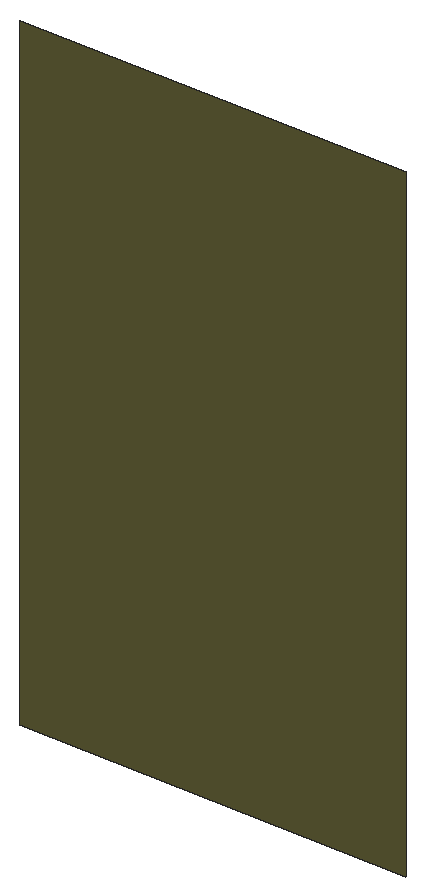
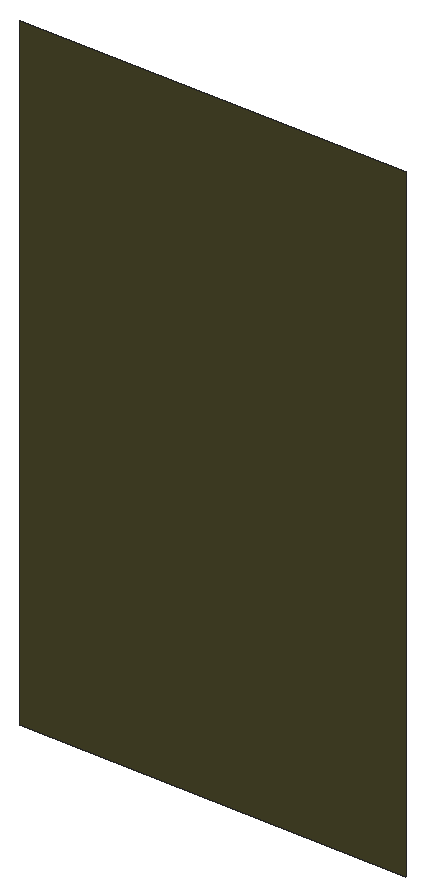
# SketchUp Ruby script. Lengths in inches.
U = 1.inch
M = Sketchup.active_model
def pt(a) = Geom::Point3d.new(a.map { |v| v * U })
def face(e, loops, mat)
  f = e.add_face(loops[0].map { |a| pt(a) })
  loops[1..].each { |l| e.add_face(l.map { |a| pt(a) }).erase! }
  f.material = f.back_material = mat if mat
  f
end
# faces: each face lists its corners as indices into pts; further lists are holes
def faces(e, pts, list, mat = nil) = list.each { |f| face(e, (f[0].is_a?(Array) ? f : [f]).map { |l| l.map { |i| pts[i] } }, mat) }
# xy, xz, yz: faces in a plane at the given z, y or x. An outline is a flat list of corners, or four numbers for a rectangle; further outlines are holes
def ring(l) = l.size == 4 ? [[l[0], l[1]], [l[2], l[1]], [l[2], l[3]], [l[0], l[3]]] : l.each_slice(2).to_a
def flat(e, list, mat, &to3) = list.each { |f| face(e, (f[0].is_a?(Array) ? f : [f]).map { |l| ring(l).map { |u, v| to3.(u, v) } }, mat) }
def xy(e, z, list, mat = nil) = flat(e, list, mat) { |x, y| [x, y, z] }
def xz(e, y, list, mat = nil) = flat(e, list, mat) { |x, z| [x, y, z] }
def yz(e, x, list, mat = nil) = flat(e, list, mat) { |y, z| [x, y, z] }
def lines(e, pts, list) = list.each { |a, b| e.add_line(pt(pts[a]), pt(pts[b])) }
# prism: a flat outline (further loops are holes) pulled along v
def prism(e, loops, v, mat = nil)
  f = face(e, loops, mat); d = Geom::Vector3d.new(v.map { |x| x * U })
  f.pushpull(f.normal.samedirection?(d) ? d.length : -d.length)
end
def box(e, o, s, mat = nil) = prism(e, [[o, [o[0] + s[0], o[1], o[2]], [o[0] + s[0], o[1] + s[1], o[2]], [o[0], o[1] + s[1], o[2]]]], [0, 0, s[2]], mat)
def at(x, y, z, deg = 0) = Geom::Transformation.translation(pt([x, y, z])) * Geom::Transformation.rotation(ORIGIN, Z_AXIS, deg.degrees)
def axes(o, x, y, z) = Geom::Transformation.new([*x, 0, *y, 0, *z, 0, *pt(o).to_a, 1])
def part(name) = M.definitions.add(name)
# library, detail: a bought-in or finely detailed component or shape, given as its bounding box
def library(name, o, s) = part(name).tap { |d| box(d.entities, o, s) }
def detail(e, o, s) = box(e.add_group.entities, o, s)
def put(e, d, t, mat = nil) = e.add_instance(d, t).tap { |i| i.material = mat if mat }
def group(e, t, mat = nil) = e.add_group.tap { |g| g.transformation = t; g.material = mat if mat }.entities
root = M.entities
M.materials.add("[0057_DarkKhaki]").color = [96, 93, 54]
xz(root,223.5,[[11.875,0,111.625,163.5625]],"[0057_DarkKhaki]")
